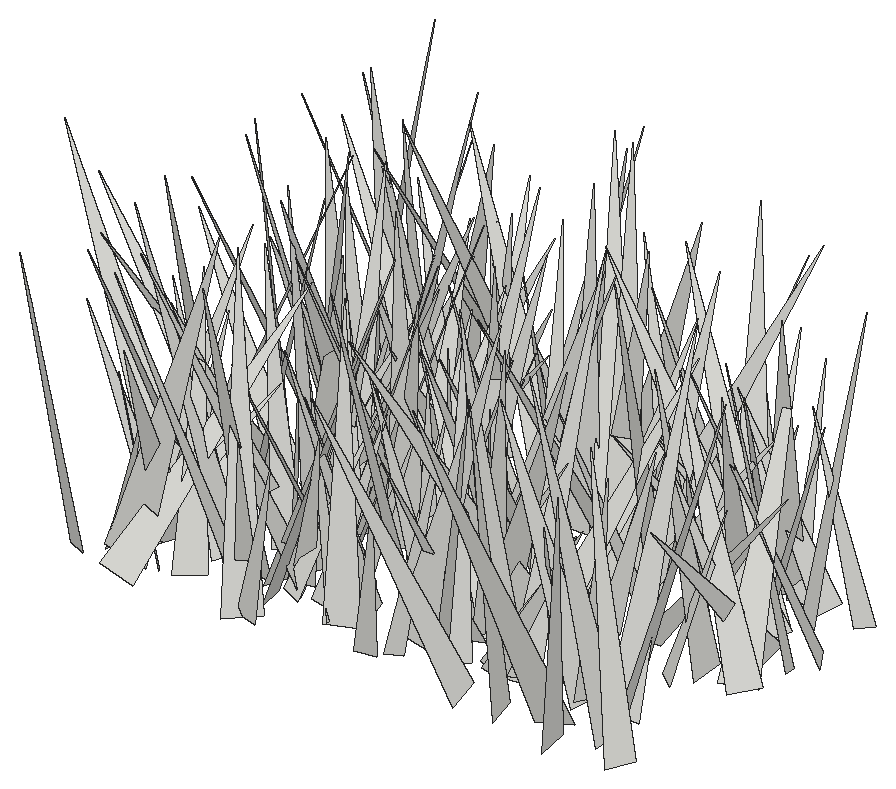
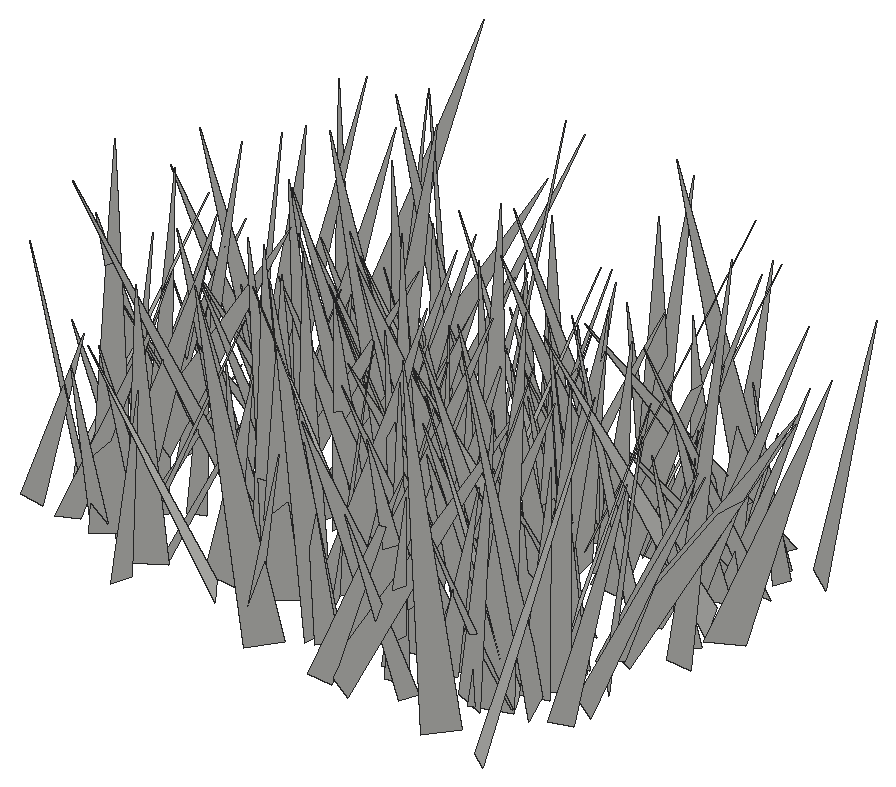
# SketchUp Ruby script. Lengths in inches.
U = 1.inch
M = Sketchup.active_model
def pt(a) = Geom::Point3d.new(a.map { |v| v * U })
def face(e, loops, mat)
  f = e.add_face(loops[0].map { |a| pt(a) })
  loops[1..].each { |l| e.add_face(l.map { |a| pt(a) }).erase! }
  f.material = f.back_material = mat if mat
  f
end
# faces: each face lists its corners as indices into pts; further lists are holes
def faces(e, pts, list, mat = nil) = list.each { |f| face(e, (f[0].is_a?(Array) ? f : [f]).map { |l| l.map { |i| pts[i] } }, mat) }
# xy, xz, yz: faces in a plane at the given z, y or x. An outline is a flat list of corners, or four numbers for a rectangle; further outlines are holes
def ring(l) = l.size == 4 ? [[l[0], l[1]], [l[2], l[1]], [l[2], l[3]], [l[0], l[3]]] : l.each_slice(2).to_a
def flat(e, list, mat, &to3) = list.each { |f| face(e, (f[0].is_a?(Array) ? f : [f]).map { |l| ring(l).map { |u, v| to3.(u, v) } }, mat) }
def xy(e, z, list, mat = nil) = flat(e, list, mat) { |x, y| [x, y, z] }
def xz(e, y, list, mat = nil) = flat(e, list, mat) { |x, z| [x, y, z] }
def yz(e, x, list, mat = nil) = flat(e, list, mat) { |y, z| [x, y, z] }
def lines(e, pts, list) = list.each { |a, b| e.add_line(pt(pts[a]), pt(pts[b])) }
# prism: a flat outline (further loops are holes) pulled along v
def prism(e, loops, v, mat = nil)
  f = face(e, loops, mat); d = Geom::Vector3d.new(v.map { |x| x * U })
  f.pushpull(f.normal.samedirection?(d) ? d.length : -d.length)
end
def box(e, o, s, mat = nil) = prism(e, [[o, [o[0] + s[0], o[1], o[2]], [o[0] + s[0], o[1] + s[1], o[2]], [o[0], o[1] + s[1], o[2]]]], [0, 0, s[2]], mat)
def at(x, y, z, deg = 0) = Geom::Transformation.translation(pt([x, y, z])) * Geom::Transformation.rotation(ORIGIN, Z_AXIS, deg.degrees)
def axes(o, x, y, z) = Geom::Transformation.new([*x, 0, *y, 0, *z, 0, *pt(o).to_a, 1])
def part(name) = M.definitions.add(name)
# library, detail: a bought-in or finely detailed component or shape, given as its bounding box
def library(name, o, s) = part(name).tap { |d| box(d.entities, o, s) }
def detail(e, o, s) = box(e.add_group.entities, o, s)
def put(e, d, t, mat = nil) = e.add_instance(d, t).tap { |i| i.material = mat if mat }
def group(e, t, mat = nil) = e.add_group.tap { |g| g.transformation = t; g.material = mat if mat }.entities
root = M.entities
c1 = part("fur_instance\#9")
p = [[0.8125,0,1.79],[0.67,-0.02,1.48],[0,-0.11,0],[0,0.11,0]]
faces(c1.entities,p,[[0,1,2,3]])
put(root,c1,axes([478.91,6.48,-21.86],[0.82289,-7.98079,0.80674],[-7.83354,-0.97405,-1.64552],[-1.72608,0.61581,7.85254]))
put(root,c1,axes([474.97,6,-21.86],[-6.88482,-1.0416,0.48285],[-0.90858,6.73783,1.57954],[0.70182,-1.49517,6.78165]))
put(root,c1,axes([479.84,5.16,-21.86],[5.74214,0.07937,1.80023],[0.34922,-5.94743,-0.85168],[-1.76782,-0.91707,5.67918]))
put(root,c1,axes([465.11,5.5,-21.86],[0.44262,-3.83329,1.02735],[-3.85493,-0.16968,1.02773],[0.94293,1.1057,3.71938]))
put(root,c1,axes([464.32,6.58,-21.86],[3.06057,-3.28635,0.3748],[-3.27189,-3.08287,-0.31361],[-0.4851,0.05914,4.47983]))
put(root,c1,axes([470.19,6.19,-21.86],[1.46502,-3.697,0.60293],[-3.73698,-1.39797,0.50827],[0.25762,0.74531,3.94408]))
put(root,c1,axes([476.87,5.85,-21.86],[-6.1633,-1.76581,2.36846],[-1.74431,6.59751,0.37966],[2.38433,0.26209,6.40002]))
put(root,c1,axes([456.92,5.8125,-21.86],[-3.28868,-4.79968,1.75844],[-5.10998,3.14053,-0.98472],[0.13097,2.01112,5.73434]))
put(root,c1,axes([464.55,6.37,-21.86],[-6.31151,-2.93767,0.11387],[-2.9284,6.25835,-0.85765],[-0.25951,0.82534,6.90866]))
put(root,c1,axes([459.37,8.6,-21.86],[4.65411,-4.15615,0.09318],[-4.0063,-4.52139,-1.56511],[-1.10988,-1.10744,6.04026]))
put(root,c1,axes([472.78,7.4,-21.86],[4.65665,4.64477,2.8893],[5.46904,-4.02795,-2.33914],[-0.10763,-3.71592,6.14709]))
put(root,c1,axes([458.74,6.38,-21.86],[0.11593,7.32982,3.76994],[7.80213,1.11829,-2.4142],[2.6581,-3.60212,6.9218]))
put(root,c1,axes([457.89,6.84,-21.86],[3.70802,-0.97097,0.29213],[-0.94384,-3.70994,-0.3508],[-0.37053,-0.26665,3.81695]))
put(root,c1,axes([482.79,5.47,-21.86],[-5.69821,2.17721,0.97614],[2.15034,5.78116,-0.34192],[1.034,-0.02439,6.0904]))
put(root,c1,axes([463.35,8.4,-21.86],[-1.28259,-7.19659,1.19017],[-7.23451,1.40948,0.72639],[0.93233,1.03678,7.27381]))
put(root,c1,axes([464.96,5.48,-21.86],[-5.4488,4.52209,1.619],[4.59694,5.6194,-0.22458],[1.39234,-0.85616,7.07731]))
put(root,c1,axes([481.26,6.75,-21.86],[-7.32255,-0.11088,1.35528],[-0.08815,7.44603,0.13288],[1.35695,-0.11461,7.32218]))
put(root,c1,axes([460.31,6.38,-21.86],[-3.16034,-1.96863,0.75138],[-2.10046,2.8354,-1.40585],[-0.16774,1.5852,3.44773]))
put(root,c1,axes([465.29,8.85,-21.86],[-6.90561,-3.33755,0.10935],[-3.32242,6.89219,0.54573],[0.33571,-0.44394,7.65042]))
put(root,c1,axes([469.93,9.27,-21.86],[-6.44031,-4.10602,1.97316],[-3.85542,6.73281,1.42663],[2.42663,-0.20036,7.50344]))
put(root,c1,axes([478.85,8.51,-21.86],[-6.00437,2.1113,1.91932],[2.55574,5.96789,1.43049],[1.26869,-2.0299,6.20191]))
put(root,c1,axes([474.82,7.91,-21.86],[1.91277,-3.82749,0.78831],[-3.61325,-1.39793,1.9799],[1.48846,1.5251,3.7932]))
put(root,c1,axes([468.26,7.23,-21.86],[-2.20554,5.93145,2.00046],[6.2413,2.24627,0.22087],[0.47966,-1.95462,6.32437]))
put(root,c1,axes([470.98,8,-21.86],[1.45839,-7.20301,2.88114],[-7.56056,-0.66269,2.17028],[1.73849,3.16049,7.02141]))
put(root,c1,axes([472.81,9.44,-21.86],[-0.13118,-4.53208,0.33432],[-4.41868,0.04908,-1.06843],[-1.06148,0.35576,4.40629]))
put(root,c1,axes([463.24,7.625,-21.86],[-7.48937,-0.81173,0.36322],[-0.84224,7.4632,-0.68756],[0.28542,0.72333,7.50179]))
put(root,c1,axes([465.13,8.83,-21.86],[1.90373,-3.64825,0.45227],[-3.65968,-1.83258,0.622],[0.34793,0.68584,4.0678]))
put(root,c1,axes([461.44,6.78,-21.86],[-4.06626,4.25963,1.22614],[4.27905,4.20638,-0.4224],[1.15655,-0.5867,5.87371]))
put(root,c1,axes([468.56,8.82,-21.86],[-5.39834,-1.72938,0.70035],[-1.70183,5.44274,0.32197],[0.76486,-0.09564,5.65943]))
put(root,c1,axes([476.72,9.35,-21.86],[-1.23844,-4.00226,0.78585],[-3.84524,1.41955,1.16979],[1.36007,0.36904,4.02286]))
put(root,c1,axes([459.12,8.45,-21.86],[-4.89818,0.93846,0.55806],[1.01529,4.8584,0.74127],[0.40164,-0.83642,4.93188]))
put(root,c1,axes([474.54,8.14,-21.86],[1.50617,-3.93782,1.16858],[-3.70084,-0.76096,2.20573],[1.78207,1.74788,3.59301]))
put(root,c1,axes([475.43,8.18,-21.86],[0.00148,-6.83986,3.17541],[-7.42007,-0.56775,-1.21947],[-1.34516,3.12424,6.73027]))
put(root,c1,axes([466.74,9.63,-21.86],[-2.68226,-4.58353,0.12394],[-4.53778,2.63294,-0.83358],[-0.65781,0.52677,5.24485]))
put(root,c1,axes([464.9,7.23,-21.86],[6.72772,1.76518,0.89994],[1.69777,-6.77807,0.60273],[-1.02144,0.36032,6.92927]))
put(root,c1,axes([459.32,5.11,-21.86],[-1.44675,6.62808,0.1342],[5.91861,1.35324,-3.03008],[2.98656,0.529,6.06986]))
put(root,c1,axes([478.81,8.51,-21.86],[4.38951,-2.01268,1.547],[-2.15257,-4.58905,0.13732],[-1.34555,0.7756,4.82698]))
put(root,c1,axes([466.71,8.05,-21.86],[-0.11814,4.24138,1.60816],[4.31681,0.59918,-1.26317],[1.39308,-1.49704,4.05064]))
put(root,c1,axes([467.78,7.41,-21.86],[-4.50739,-0.00087,0.31518],[-0.09503,4.31184,-1.34718],[0.30051,1.35052,4.30136]))
put(root,c1,axes([471.07,6.77,-21.86],[-4.41847,1.33903,1.10997],[0.76139,4.21375,-2.05244],[1.56375,1.73183,4.13562]))
put(root,c1,axes([459.41,10.42,-21.86],[-2.8111,-5.64649,0.53318],[-5.64839,2.7334,-0.83291],[-0.51273,0.84565,6.25232]))
put(root,c1,axes([474.81,11.52,-21.86],[1.75618,-7.20882,1.45322],[-6.25973,-2.24953,-3.59425],[-3.85938,0.3683,6.49097]))
put(root,c1,axes([465.3,7.91,-21.86],[1.23248,3.89294,0.26564],[3.83774,-1.15903,-0.82034],[0.70519,-0.49622,4.00013]))
put(root,c1,axes([470.73,9.59,-21.86],[-5.18821,0.426,1.12668],[0.56814,5.25845,0.62796],[1.06213,-0.73187,5.16766]))
put(root,c1,axes([473.26,7.64,-21.86],[-5.70691,2.72816,1.15825],[2.57005,5.80682,-1.01437],[1.47624,0.43731,6.24361]))
put(root,c1,axes([461.66,8.68,-21.86],[-4.99004,2.24313,0.58277],[2.2784,5.00139,0.2583],[0.42444,-0.4756,5.46492]))
put(root,c1,axes([467.48,10.19,-21.86],[-3.54687,-2.63553,0.56126],[-2.61948,3.58991,0.30355],[0.63194,0.08835,4.40842]))
put(root,c1,axes([458.45,7.59,-21.86],[-0.23722,4.19444,0.05409],[3.55446,0.22976,-2.22834],[2.22756,0.08005,3.56147]))
put(root,c1,axes([460.93,8.72,-21.86],[-3.32365,-1.7064,1.24939],[-2.04417,3.18881,-1.08271],[0.54234,1.56176,3.57578]))
put(root,c1,axes([462.51,11.34,-21.86],[2.04194,-5.37013,1.21962],[-4.97283,-2.35693,-2.05211],[-2.36574,0.31918,5.36625]))
put(root,c1,axes([467.51,8.93,-21.86],[3.08965,-1.86478,1.07968],[-2.12915,-2.93231,1.02827],[-0.33144,1.45368,3.45919]))
put(root,c1,axes([472.77,10.27,-21.86],[5.91489,-2.56905,1.81184],[-2.61095,-6.16477,-0.21752],[-1.75092,0.51416,6.44505]))
put(root,c1,axes([472.59,10.71,-21.86],[5.68552,-4.38043,0.51347],[-4.40819,-5.61738,0.88871],[0.14016,1.01677,7.12204]))
put(root,c1,axes([463.87,9.87,-21.86],[1.95949,2.80373,1.45551],[3.04239,-2.136,0.01872],[-0.85045,-1.18135,3.42055]))
put(root,c1,axes([458.74,9.42,-21.86],[1.07751,-3.9043,2.33703],[-4.53898,-0.75293,0.83488],[0.32078,2.46086,3.96327]))
put(root,c1,axes([464.26,8.3,-21.86],[6.79493,0.95964,1.40947],[0.56386,-6.72962,1.86359],[-1.60922,1.6941,6.60447]))
put(root,c1,axes([464.94,10.01,-21.86],[4.01633,-1.15722,1.23996],[-1.33038,-4.12648,0.45808],[-1.05202,0.80037,4.15454]))
put(root,c1,axes([457.95,8.09,-21.86],[1.29367,6.30142,0.29631],[6.29029,-1.26564,-0.54746],[0.47747,-0.39942,6.4095]))
put(root,c1,axes([480.79,8.125,-21.86],[5.94248,2.0649,1.47313],[1.51819,-5.90154,2.14801],[-2.032,1.62942,5.91295]))
put(root,c1,axes([480.52,8.37,-21.86],[0.44326,7.59594,0.73525],[7.62112,-0.4789,0.35297],[-0.39679,-0.71255,7.60067]))
put(root,c1,axes([465.1875,10.35,-21.86],[6.72571,2.73267,0.89443],[2.78268,-6.75899,-0.27437],[-0.72399,-0.59256,7.25447]))
put(root,c1,axes([471.07,11.1875,-21.86],[3.3459,3.39415,0.39754],[3.18536,-2.89609,-2.08314],[1.23764,-1.72213,4.2867]))
put(root,c1,axes([470,9.55,-21.86],[5.23362,2.8594,0.35445],[2.818,-5.23298,0.60609],[-0.60055,0.36375,5.93293]))
put(root,c1,axes([473.15,10.32,-21.86],[-3.6214,4.75768,0.36392],[4.63089,3.39426,1.70771],[-1.15013,-1.31374,5.73008]))
put(root,c1,axes([472.12,12.93,-21.86],[0.31088,-6.10314,0.84199],[-6.04835,-0.46277,-1.12122],[-1.17245,0.76905,6.00731]))
put(root,c1,axes([463.07,10.53,-21.86],[-1.86081,5.49202,1.44787],[5.66351,1.67938,0.90859],[-0.42807,-1.65488,5.72707]))
put(root,c1,axes([469.125,11.37,-21.86],[4.20297,-1.11156,0.80651],[-1.18233,-4.24977,0.30429],[-0.69867,0.5049,4.33681]))
put(root,c1,axes([476.14,8.05,-21.86],[1.42623,8.08681,0.06748],[7.92603,-1.41139,1.61901],[-1.60595,0.21606,8.05043]))
put(root,c1,axes([456.97,14.03,-21.86],[-2.27672,-7.40144,1.23154],[-7.29478,2.48469,1.44709],[1.75622,0.72557,7.60728]))
put(root,c1,axes([467.48,13.25,-21.86],[-5.5722,-4.07145,0.43281],[-4.071,5.58734,0.1482],[0.43699,0.13539,6.89957]))
put(root,c1,axes([468.92,11.79,-21.86],[4.42426,3.38365,0.88099],[3.49585,-4.30744,-1.01209],[-0.06566,-1.34021,5.47712]))
put(root,c1,axes([456.66,11.72,-21.86],[-5.80896,4.38047,0.69826],[4.41604,5.60261,1.59041],[-0.41794,-1.68592,7.09952]))
put(root,c1,axes([468.05,12.1,-21.86],[-2.1087,-2.96786,0.97974],[-3.12443,1.97245,-0.74971],[-0.07759,1.23123,3.56269]))
put(root,c1,axes([464.12,10.89,-21.86],[-6.95078,-0.2098,1.40903],[-0.48679,6.94525,-1.36721],[1.33881,1.43604,6.81821]))
put(root,c1,axes([481.99,15.39,-21.86],[4.40481,-2.70951,0.82389],[-1.71706,-3.76665,-3.20728],[-2.2521,-2.42766,4.05674]))
put(root,c1,axes([480.11,11.52,-21.86],[2.28219,3.09258,0.57784],[3.14608,-2.24088,-0.43237],[0.01087,-0.72161,3.81909]))
put(root,c1,axes([480.92,12.9,-21.86],[-6.33484,-0.15602,2.15214],[0.09289,6.64883,0.75543],[2.15578,-0.74496,6.29157]))
put(root,c1,axes([472.11,14.46,-21.86],[-0.6438,-6.00502,0.1729],[-5.98541,0.62626,-0.53591],[-0.51472,0.22839,6.0156]))
put(root,c1,axes([460.02,12.36,-21.86],[-5.05806,4.73106,0.08976],[4.36112,4.60989,2.7757],[-1.83619,-2.08349,6.34527]))
put(root,c1,axes([457.41,12.78,-21.86],[1.8239,-3.22944,0.77362],[-3.28665,-1.6292,0.94764],[0.47508,1.1273,3.58579]))
put(root,c1,axes([469.51,12.19,-21.86],[-4.422,-0.95671,1.75223],[-1.16644,4.69405,-0.38074],[1.6202,0.76828,4.50826]))
put(root,c1,axes([471.46,11.85,-21.86],[2.90611,1.79436,1.69144],[1.585,-3.36196,0.84331],[-1.88904,-0.06039,3.30969]))
put(root,c1,axes([466.53,13.26,-21.86],[2.05152,-6.96349,2.48946],[-7.36809,-2.14532,0.07104],[-0.63146,2.40909,7.25905]))
put(root,c1,axes([464.59,13.24,-21.86],[3.14021,-1.95272,0.11029],[-1.95573,-3.13292,0.21476],[0.01996,0.24059,3.6916]))
put(root,c1,axes([465.5,14.2,-21.86],[0.26156,-6.27199,1.2943],[-6.21893,0.06053,1.55008],[1.52905,1.31908,6.08306]))
put(root,c1,axes([467.56,13.21,-21.86],[2.21811,-2.97156,1.30139],[-3.14682,-2.35396,-0.01147],[-0.78819,1.03561,3.7081]))
put(root,c1,axes([459.17,14.88,-21.86],[-0.73144,-5.99959,0.26703],[-5.39662,0.53861,-2.681],[-2.63493,0.56233,5.41685]))
put(root,c1,axes([481.93,14.02,-21.86],[-4.18916,1.41328,1.44955],[1.84035,4.04661,1.3732],[0.84361,-1.80976,4.20247]))
put(root,c1,axes([476.04,13.1875,-21.86],[1.31447,-3.85278,1.5031],[-4.0825,-0.95693,1.11736],[0.66058,1.75255,3.91449]))
put(root,c1,axes([462.54,13.49,-21.86],[2.46707,-3.42013,1.11602],[-3.59628,-2.30764,0.87798],[0.09798,1.4166,4.12467]))
put(root,c1,axes([464.01,13,-21.86],[2.76185,-3.07557,2.49035],[-3.57907,-3.23702,-0.02845],[-1.68858,1.83068,4.13354]))
put(root,c1,axes([482.87,12.72,-21.86],[-3.78677,4.88862,0.77178],[4.90876,3.58599,1.37062],[-0.63111,-1.44081,6.0299]))
put(root,c1,axes([464.23,14.19,-21.86],[2.06201,-3.51619,0.27094],[-3.44771,-1.94389,1.0117],[0.74186,0.73932,3.94867]))
put(root,c1,axes([458.03,10.8,-21.86],[6.85876,3.23862,0.41321],[3.02392,-6.66397,2.03701],[-1.23097,1.67477,7.30628]))
put(root,c1,axes([469.53,12.39,-21.86],[5.50822,-3.47682,2.75588],[-4.25576,-5.38219,1.71589],[-1.25366,2.99458,6.28367]))
put(root,c1,axes([459.06,13.66,-21.86],[6.14666,2.4589,1.36982],[2.59506,-6.2248,-0.47069],[-1.09008,-0.95377,6.60349]))
put(root,c1,axes([475.91,15.42,-21.86],[-4.5248,-1.88356,0.71077],[-1.69814,4.51006,1.14127],[1.08134,-0.799,4.76646]))
put(root,c1,axes([477.82,13.39,-21.86],[3.92135,-2.35365,0.03406],[-2.05535,-3.39138,2.27856],[1.14733,1.96892,3.96545]))
put(root,c1,axes([470.03,10.6875,-21.86],[-7.05102,3.6652,1.50452],[2.87345,6.84526,-3.20935],[2.72774,2.26338,7.26985]))
put(root,c1,axes([467.76,12.31,-21.86],[-0.62554,4.99616,0.12365],[4.99768,0.62512,0.02455],[-0.009,-0.12574,5.03511]))
put(root,c1,axes([475.21,15.99,-21.86],[-1.63485,-6.2778,0.46595],[-5.97391,1.39539,-2.16005],[-1.98499,0.97094,6.117]))
put(root,c1,axes([473.99,12.6,-21.86],[1.01067,5.88602,0.15693],[5.68933,-0.93518,-1.56469],[1.51703,-0.41415,5.76354]))
put(root,c1,axes([462.57,15.13,-21.86],[4.49175,-3.99144,0.42922],[-3.97143,-4.32409,1.3497],[0.58618,1.28931,5.8554]))
put(root,c1,axes([468.29,16.01,-21.86],[6.0824,-3.06076,1.36011],[-2.97573,-6.23245,-0.71791],[-1.53726,-0.04598,6.77115]))
put(root,c1,axes([475.52,16.75,-21.86],[-6.68782,-2.79113,3.18251],[-2.04813,7.34131,2.13449],[3.70459,-0.98003,6.92541]))
put(root,c1,axes([460.86,17.75,-21.86],[1.6119,-7.35068,0.1441],[-7.34568,-1.61634,-0.28263],[-0.30696,0.08011,7.52003]))
put(root,c1,axes([477.9,16.28,-21.86],[0.30074,-4.21199,0.28121],[-4.14735,-0.24225,0.80695],[0.78703,0.33293,4.14489]))
put(root,c1,axes([466.3,17.8125,-21.86],[4.06405,-3.6671,0.18626],[-3.28339,-3.75381,-2.26428],[-1.64366,-1.56845,4.98369]))
put(root,c1,axes([483.65,16.23,-21.86],[-5.39414,-3.77764,0.22745],[-3.78403,5.38986,-0.22257],[0.05845,0.31282,6.58162]))
put(root,c1,axes([479.16,17.27,-21.86],[6.03542,-2.39463,0.80521],[-2.12324,-5.9379,-1.74415],[-1.3691,-1.34759,6.25448]))
put(root,c1,axes([476.52,15.5625,-21.86],[3.53808,2.09554,0.91862],[2.27584,-3.39762,-1.01485],[-0.23603,-1.34836,3.98489]))
put(root,c1,axes([464.96,12.31,-21.86],[5.4592,3.52611,0.65952],[3.05756,-5.20187,2.50265],[-1.87611,1.78282,5.99776]))
put(root,c1,axes([460.875,14.32,-21.86],[1.67584,3.97009,0.12724],[3.80521,-1.56498,-1.28741],[1.13936,-0.61275,4.1125]))
put(root,c1,axes([469.67,15.42,-21.86],[2.98572,-5.88102,1.99527],[-6.13329,-2.44486,1.97166],[0.97482,2.63026,6.29392]))
put(root,c1,axes([473.82,13.01,-21.86],[-2.11402,4.56513,0.60738],[3.84978,2.11854,-2.52378],[2.52756,0.59144,4.35202]))
put(root,c1,axes([459.125,15.375,-21.86],[-4.48303,2.72425,0.35571],[2.72908,4.33728,1.17718],[-0.3165,-1.18832,5.11208]))
put(root,c1,axes([459.7,16.69,-21.86],[0.9975,-5.62203,0.93729],[-5.55991,-0.75041,1.41599],[1.25425,1.14473,5.53148]))
put(root,c1,axes([482.46,12.84,-21.86],[-4.33285,5.33033,0.39838],[5.19442,4.31986,-1.30443],[1.26061,0.52067,6.74422]))
put(root,c1,axes([464.6,15.2,-21.86],[3.74419,-3.98525,0.35569],[-3.51637,-3.04515,2.89653],[1.90889,2.20738,4.63803]))
put(root,c1,axes([473.17,13.1,-21.86],[-6.61706,2.95045,0.41304],[2.75432,6.44194,-1.89112],[1.13554,1.56763,6.99387]))
put(root,c1,axes([483.23,14.91,-21.86],[-5.46466,-2.11839,0.66349],[-2.21236,5.05235,-2.09036],[-0.18243,2.18553,5.47545]))
put(root,c1,axes([469.875,14.71,-21.86],[6.41211,-0.61612,1.30158],[-0.93497,-6.2989,1.62436],[-1.09524,1.77006,6.23347]))
put(root,c1,axes([462.92,14.24,-21.86],[-0.70792,6.63222,0.94241],[6.69223,0.65809,0.39581],[-0.29764,-0.97786,6.65814]))
put(root,c1,axes([469.09,16.48,-21.86],[-4.90354,-1.85753,0.89414],[-1.8937,4.97041,-0.05944],[0.81474,0.37312,5.24324]))
put(root,c1,axes([475.28,15.85,-21.86],[3.04424,4.32162,0.01521],[3.85535,-2.70735,-2.39804],[1.95268,-1.39208,4.71097]))
put(root,c1,axes([481.16,16.33,-21.86],[-4.49913,6.58347,1.21187],[6.27218,3.63575,3.53468],[-2.33889,-2.91414,7.14775]))
put(root,c1,axes([473.88,14.89,-21.86],[0.68062,5.93772,0.86921],[5.89172,-0.495,-1.23203],[1.14003,-0.98679,5.84823]))
put(root,c1,axes([459.11,17.27,-21.86],[6.76883,1.43904,1.95286],[1.74836,-6.90673,-0.9705],[-1.68159,-1.38844,6.85171]))
put(root,c1,axes([465.9375,14.79,-21.86],[-1.59492,4.69203,0.53683],[4.53057,1.68008,-1.22409],[1.33316,-0.09626,4.80214]))
put(root,c1,axes([460.06,17.52,-21.86],[-5.59539,-3.44886,0.89561],[-3.54081,5.56848,-0.67808],[0.39927,1.05,6.53783]))
put(root,c1,axes([468.375,17.59,-21.86],[-3.68845,0.83243,0.84341],[0.99836,3.66829,0.74556],[0.6384,-0.92717,3.70698]))
put(root,c1,axes([476.71,19.6,-21.86],[-4.21387,-1.59887,0.24339],[-1.27519,3.70248,2.24451],[0.99474,-2.02671,3.90836]))
put(root,c1,axes([475.46,16.05,-21.86],[-1.23701,6.48468,1.94316],[6.59867,1.59608,-1.12573],[1.51147,-1.6609,6.50492]))
put(root,c1,axes([478.79,19.44,-21.86],[-1.94792,-5.41513,0.85515],[-5.11405,2.12183,1.78705],[1.97517,0.15336,5.47032]))
put(root,c1,axes([458.23,16.67,-21.86],[-4.69579,-3.74143,2.09942],[-4.25802,4.44495,-1.60248],[0.52452,2.58851,5.78625]))
put(root,c1,axes([457.69,18.72,-21.86],[-2.53227,-4.93937,0.36335],[-4.86121,2.40071,-1.24381],[-0.94765,0.88376,5.4095]))
put(root,c1,axes([479.48,19.34,-21.86],[4.02071,-6.30995,0.86141],[-6.36147,-4.02715,0.19326],[-0.29869,0.83076,7.47959]))
put(root,c1,axes([480.6,16.625,-21.86],[4.03699,1.00135,1.00845],[0.75439,-4.0837,1.03503],[-1.2044,0.79854,4.02849]))
put(root,c1,axes([469.66,18.43,-21.86],[-4.6895,-2.45579,1.69505],[-2.43913,4.97359,0.45768],[1.71894,0.35769,5.27378]))
put(root,c1,axes([480.68,16.8,-21.86],[-6.09178,4.42452,0.24879],[4.41982,6.03543,0.88707],[-0.32169,-0.86331,7.47659]))
put(root,c1,axes([478.4,19.94,-21.86],[-4.14982,-0.72477,0.23143],[-0.53834,3.70403,1.94686],[0.53763,-1.88541,3.73578]))
put(root,c1,axes([474.2,18.12,-21.86],[-3.43259,1.11019,2.13702],[1.24058,4.00441,-0.08763],[2.06406,-0.56053,3.60659]))
put(root,c1,axes([459.36,18.52,-21.86],[-4.56803,3.68378,2.77525],[4.20348,4.93276,0.37129],[1.89817,-2.05836,5.85656]))
put(root,c1,axes([460.5,17.71,-21.86],[2.21445,2.95218,0.72503],[3.03203,-2.20951,-0.26401],[-0.21871,-0.73996,3.68096]))
put(root,c1,axes([462.85,19.4375,-21.86],[0.6809,-4.24063,0.83858],[-4.19337,-0.85411,-0.91428],[-1.04966,0.66131,4.19651]))
put(root,c1,axes([474.35,16.57,-21.86],[2.96543,7.80813,0.73471],[7.53088,-2.61577,-2.59693],[2.18919,-1.57838,7.9383]))
put(root,c1,axes([457.58,20.21,-21.86],[3.46395,-3.11936,0.86631],[-2.7787,-3.51575,-1.54862],[-1.66124,-0.62369,4.39672]))
put(root,c1,axes([471.4,19.3,-21.86],[2.15737,-6.51602,1.69287],[-6.69271,-1.88316,1.28061],[0.7294,1.99342,6.74336]))
put(root,c1,axes([470.8,18.26,-21.86],[-0.16128,6.84934,2.86842],[7.42417,0.20732,-0.07764],[0.15166,-2.86546,6.8508]))
put(root,c1,axes([464.875,16.32,-21.86],[-4.26385,3.34064,0.29483],[3.15748,4.15963,-1.468],[1.13011,0.98225,5.21395]))
put(root,c1,axes([481.48,19.38,-21.86],[-4.32688,2.05759,1.06704],[2.30248,4.07514,1.47851],[0.2661,-1.80382,4.55737]))
put(root,c1,axes([470.11,17.94,-21.86],[-7.19785,3.45896,0.52945],[3.49375,7.17168,0.64382],[0.19618,-0.81015,7.95983]))
put(root,c1,axes([462.97,16.14,-21.86],[7.1916,2.06862,2.54607],[1.20326,-7.37063,2.58975],[-3.05186,1.96861,7.0208]))
put(root,c1,axes([478.32,18.5,-21.86],[3.72364,-1.08643,0.80362],[-1.21362,-3.72465,0.58799],[-0.59435,0.79892,3.83407]))
put(root,c1,axes([464.55,18.2,-21.86],[-5.71185,4.45959,0.23835],[4.39877,5.55102,1.55146],[-0.77178,-1.36683,7.07857]))
put(root,c1,axes([465.5,19.53,-21.86],[0.07384,-6.03784,2.03973],[-6.28438,0.27016,1.02718],[1.05955,2.02311,5.95028]))
put(root,c1,axes([478.22,19.12,-21.86],[-5.88175,-1.50758,0.15009],[-1.51502,5.85044,-0.60606],[-0.00586,0.62434,6.04156]))
put(root,c1,axes([464.97,18.18,-21.86],[-7.75285,-2.01113,0.68817],[-2.11722,7.53738,-1.82488],[0.1887,1.94117,7.79879]))
put(root,c1,axes([472.87,18.01,-21.86],[-1.87564,7.62096,1.95831],[7.8685,1.80971,0.49369],[-0.027,-2.0194,7.83284]))
put(root,c1,axes([460.66,18.68,-21.86],[4.54931,-2.96003,1.24819],[-3.21199,-4.22741,1.68171],[-0.05363,2.09362,5.16041]))
put(root,c1,axes([483.35,19.18,-21.86],[-1.35537,3.98703,1.26023],[4.07237,0.95801,1.34893],[-0.94888,-1.58348,3.98921]))
put(root,c1,axes([463.18,18.72,-21.86],[0.71966,5.69009,1.64056],[5.43341,0.02279,-2.46251],[2.35511,-1.79132,5.17987]))
put(root,c1,axes([468.93,16.98,-21.86],[-5.00496,1.9066,1.35129],[1.19771,4.83542,-2.3864],[2.00664,1.8693,4.79477]))
put(root,c1,axes([469.59,16.34,-21.86],[5.51307,6.12337,0.96272],[5.81555,-5.55551,2.03274],[-2.14519,0.67601,7.98483]))
put(root,c1,axes([459.59,19.24,-21.86],[1.73924,-4.25815,2.51532],[-4.74882,-2.1825,-0.41111],[-1.38108,2.14207,4.58125]))
put(root,c1,axes([481.52,18.1,-21.86],[3.26782,5.25044,1.3347],[5.28581,-3.43164,0.55786],[-1.18691,-0.82697,6.1591]))
put(root,c1,axes([472.49,17.88,-21.86],[-5.1988,6.07272,1.14347],[6.1224,5.26442,-0.12263],[0.83765,-0.78798,7.99315]))
put(root,c1,axes([460.29,20.95,-21.86],[2.83404,-7.21043,2.36501],[-7.48804,-3.06648,-0.37599],[-1.22999,2.05469,7.73827]))
put(root,c1,axes([466.48,22.18,-21.86],[-0.7633,-7.78268,1.04828],[-7.63293,0.4877,-1.93706],[-1.84592,1.20152,7.57632]))
put(root,c1,axes([464.27,21.49,-21.86],[-0.22733,-5.68785,1.31588],[-5.73337,0.46581,1.02292],[1.10075,1.2515,5.59972]))
put(root,c1,axes([468.15,20.83,-21.86],[3.13443,-2.25979,0.73802],[-2.32723,-3.16608,0.18952],[-0.4851,0.5876,3.85946]))
put(root,c1,axes([459.98,19.75,-21.86],[5.69643,3.12279,1.00252],[3.16084,-5.76326,-0.00802],[-0.87518,-0.48903,6.49623]))
put(root,c1,axes([480.1875,19.13,-21.86],[0.35019,4.61175,0.40741],[4.56098,-0.41379,0.76359],[-0.79477,-0.34263,4.56155]))
put(root,c1,axes([465.74,18.71,-21.86],[-2.14385,5.53708,0.23418],[5.53457,2.15208,-0.21752],[0.2875,-0.13964,5.93364]))
put(root,c1,axes([474.15,19.58,-21.86],[-1.56415,5.71782,0.81541],[5.62888,1.31989,1.54221],[-1.29382,-1.17019,5.72377]))
put(root,c1,axes([468.69,20.41,-21.86],[7.07212,-1.1156,2.41076],[-1.38462,-7.39913,0.63784],[-2.26697,1.03896,7.1311]))
put(root,c1,axes([461.21,21.07,-21.86],[1.62899,5.48386,2.82302],[6.01922,-2.05055,0.50999],[-1.34582,-2.53344,5.69792]))
put(root,c1,axes([463.06,20.28,-21.86],[-4.64621,2.31988,0.55706],[2.32982,4.67441,-0.03457],[0.51391,-0.21773,5.19306]))
put(root,c1,axes([465.91,22.97,-21.86],[-2.5504,-6.61055,0.06946],[-6.29815,2.40698,-2.17909],[-2.00934,0.84606,6.74207]))
put(root,c1,axes([459.875,20.56,-21.86],[1.33461,3.80482,0.72121],[3.71713,-1.04467,-1.36733],[1.08616,-1.09999,3.79319]))
put(root,c1,axes([459.1,19.74,-21.86],[7.33246,2.99097,2.42144],[2.72494,-7.71469,1.27771],[-2.71735,0.33456,7.81527]))
put(root,c1,axes([458.24,24.22,-21.86],[-4.76858,-5.56642,0.65425],[-5.40433,4.79429,1.40014],[1.48534,-0.42682,7.19472]))
put(root,c1,axes([477,20.3,-21.86],[-3.82919,5.78151,1.38736],[5.88668,3.91838,-0.08139],[0.83523,-1.11076,6.93412]))
put(root,c1,axes([464.94,20.87,-21.86],[-1.18349,4.29439,0.91251],[4.36217,1.04349,0.74676],[-0.49586,-1.06979,4.39144]))
put(root,c1,axes([469.85,22.34,-21.86],[4.01839,-5.64573,1.18023],[-5.73753,-3.76564,1.52164],[0.58986,1.83314,6.76065]))
put(root,c1,axes([466.65,23.07,-21.86],[1.33499,-4.14938,1.03511],[-3.92508,-1.61935,-1.42916],[-1.69781,0.48101,4.1179]))
put(root,c1,axes([470.83,21.98,-21.86],[-3.8802,0.07929,1.10053],[0.11582,4.03064,0.11798],[1.09728,-0.14508,3.87922]))
put(root,c1,axes([463.22,22.14,-21.86],[2.09245,-2.98815,0.44058],[-2.87886,-1.81085,1.39087],[0.91397,1.13723,3.37237]))
put(root,c1,axes([476.98,21.86,-21.86],[-3.91308,1.33626,1.31278],[1.41439,4.10109,0.04154],[1.2282,-0.46546,4.13474]))
put(root,c1,axes([460.65,23.41,-21.86],[5.57249,-4.36069,0.56036],[-4.38496,-5.5781,0.19774],[-0.31889,0.50141,7.07313]))
put(root,c1,axes([473.76,20.32,-21.86],[5.03516,3.5658,0.22039],[3.50469,-5.00395,0.89105],[-0.69327,0.6016,6.10523]))
